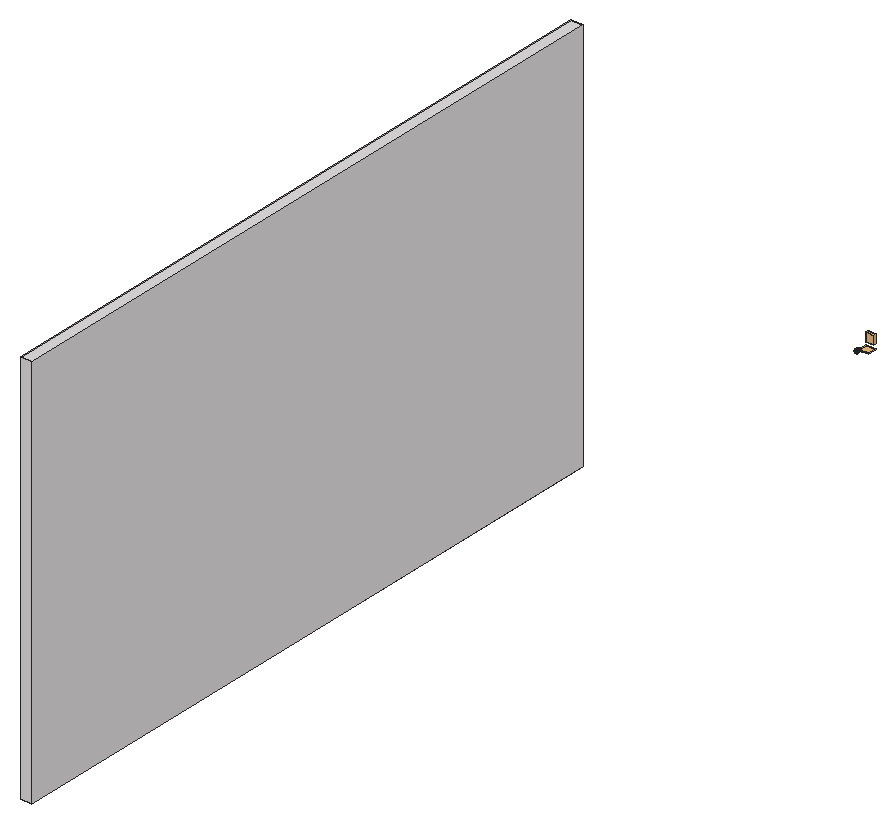
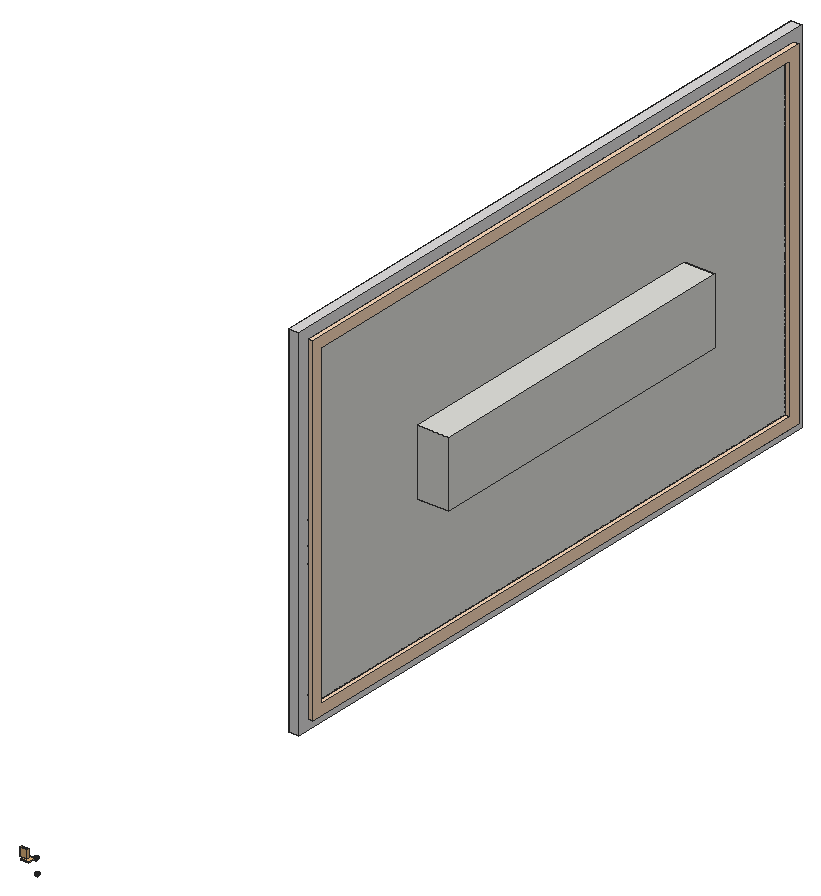
# SketchUp Ruby script. Lengths in inches.
U = 1.inch
M = Sketchup.active_model
def pt(a) = Geom::Point3d.new(a.map { |v| v * U })
def face(e, loops, mat)
  f = e.add_face(loops[0].map { |a| pt(a) })
  loops[1..].each { |l| e.add_face(l.map { |a| pt(a) }).erase! }
  f.material = f.back_material = mat if mat
  f
end
# faces: each face lists its corners as indices into pts; further lists are holes
def faces(e, pts, list, mat = nil) = list.each { |f| face(e, (f[0].is_a?(Array) ? f : [f]).map { |l| l.map { |i| pts[i] } }, mat) }
# xy, xz, yz: faces in a plane at the given z, y or x. An outline is a flat list of corners, or four numbers for a rectangle; further outlines are holes
def ring(l) = l.size == 4 ? [[l[0], l[1]], [l[2], l[1]], [l[2], l[3]], [l[0], l[3]]] : l.each_slice(2).to_a
def flat(e, list, mat, &to3) = list.each { |f| face(e, (f[0].is_a?(Array) ? f : [f]).map { |l| ring(l).map { |u, v| to3.(u, v) } }, mat) }
def xy(e, z, list, mat = nil) = flat(e, list, mat) { |x, y| [x, y, z] }
def xz(e, y, list, mat = nil) = flat(e, list, mat) { |x, z| [x, y, z] }
def yz(e, x, list, mat = nil) = flat(e, list, mat) { |y, z| [x, y, z] }
def lines(e, pts, list) = list.each { |a, b| e.add_line(pt(pts[a]), pt(pts[b])) }
# prism: a flat outline (further loops are holes) pulled along v
def prism(e, loops, v, mat = nil)
  f = face(e, loops, mat); d = Geom::Vector3d.new(v.map { |x| x * U })
  f.pushpull(f.normal.samedirection?(d) ? d.length : -d.length)
end
def box(e, o, s, mat = nil) = prism(e, [[o, [o[0] + s[0], o[1], o[2]], [o[0] + s[0], o[1] + s[1], o[2]], [o[0], o[1] + s[1], o[2]]]], [0, 0, s[2]], mat)
def at(x, y, z, deg = 0) = Geom::Transformation.translation(pt([x, y, z])) * Geom::Transformation.rotation(ORIGIN, Z_AXIS, deg.degrees)
def axes(o, x, y, z) = Geom::Transformation.new([*x, 0, *y, 0, *z, 0, *pt(o).to_a, 1])
def part(name) = M.definitions.add(name)
# library, detail: a bought-in or finely detailed component or shape, given as its bounding box
def library(name, o, s) = part(name).tap { |d| box(d.entities, o, s) }
def detail(e, o, s) = box(e.add_group.entities, o, s)
def put(e, d, t, mat = nil) = e.add_instance(d, t).tap { |i| i.material = mat if mat }
def group(e, t, mat = nil) = e.add_group.tap { |g| g.transformation = t; g.material = mat if mat }.entities
root = M.entities
M.materials.add("TV  BG light").color = [252, 218, 188]
M.materials.add("[Stone Vein Gray]").color = [225, 223, 223]
M.materials.add("green").color = [174, 139, 102]
M.materials.add("vio").color = [206, 114, 100]
c1 = part("3DGeom~250_Defintion")
p = [[-24.32,49.98,-496.93],[-31.18,-167.76,-459.32],[-244.86,-167.22,-390.18],[228.94,35.96,-443.61],[-244.86,-167.22,-390.18],[-271.06,50.6,-417.1],
  [208.38,242.18,-355.22],[-10.94,254.33,-401.4],[-271.06,50.6,-417.1],[208.38,242.18,-355.22],[-10.94,254.33,-401.4],[-29.68,-340.55,-298.625],
  [-153.05,-340.24,-258.71],[188.15,-179.91,-413.14],[-153.05,-340.24,-258.71],[-244.86,-167.22,-390.18],[420.85,12.3,-271.43],[374.59,221.7,-206.1],
  [374.59,221.7,-206.1],[208.38,242.18,-355.22],[-271.06,50.6,-417.1],[-395.65,-178.42,-224.25],[-445.17,37.67,-225.51],[-244.86,-167.22,-390.18],
  [-224.63,254.87,-332.26],[-10.94,254.33,-401.4],[-271.06,50.6,-417.1],[-224.63,254.87,-332.26],[96.95,-347.5625,-271.96],[354.35,-200.39,-264.02],
  [131.99,383.52,-171.65],[208.38,242.18,-355.22],[-10.94,254.33,-401.4],[5.36,390.53,-198.31],[-224.63,254.87,-332.26],[-240.11,-346.7,-162.91],
  [-153.05,-340.24,-258.71],[227.95,371.69,-85.56],[374.59,221.7,-206.1],[-224.63,254.87,-332.26],[-375.41,243.67,-166.34],[-118.01,390.84,-158.39],
  [-375.41,243.67,-166.34],[-153.05,-340.24,-258.71],[-29.68,-340.55,-298.625],[-20.23,-422.09,-57.92],[-29.68,-340.55,-298.625],[96.95,-347.5625,-271.96],
  [96.95,-347.5625,-271.96],[192.91,-359.39,-185.87],[192.91,-359.39,-185.87],[500,-14.65,-26.51],[354.35,-200.39,-264.02],[420.85,12.3,-271.43],
  [443.13,198.36,6],[420.85,12.3,-271.43],[420.85,12.3,-271.43],[374.59,221.7,-206.1],[422.9,-223.73,-51.92],[192.91,-359.39,-185.87],
  [354.35,-200.39,-264.02],[354.35,-200.39,-264.02],[-240.11,-346.7,-162.91],[-153.05,-340.24,-258.71],[-443.13,-198.36,-6],[-500,14.65,26.51],
  [-267.52,-358.22,-36.9],[267.52,358.22,36.9],[374.59,221.7,-206.1],[267.52,358.22,36.9],[374.59,221.7,-206.1],[227.95,371.69,-85.56],
  [20.23,422.09,57.92],[192.91,-359.39,-185.87],[232.48,-372.86,-63.41],[232.48,-372.86,-63.41],[192.91,-359.39,-185.87],[-422.9,223.73,51.92],
  [-205.0625,384.375,-62.6],[-375.41,243.67,-166.34],[-205.0625,384.375,-62.6],[-267.52,-358.22,-36.9],[-240.11,-346.7,-162.91],[267.52,358.22,36.9],
  [232.48,-372.86,-63.41],[205.0625,-384.375,62.6],[375.41,-243.67,166.34],[205.0625,-384.375,62.6],[-205.0625,384.375,-62.6],[-232.48,372.86,63.41],
  [-232.48,372.86,63.41],[-227.95,-371.69,85.56],[-267.52,-358.22,-36.9],[-131.99,-383.52,171.65],[-227.95,-371.69,85.56],[-5.36,-390.53,198.31],
  [205.0625,-384.375,62.6],[118.01,-390.84,158.39],[445.17,-37.67,225.51],[-227.95,-371.69,85.56],[395.65,178.42,224.25],[-374.59,-221.7,206.1],
  [240.11,346.7,162.91],[240.11,346.7,162.91],[267.52,358.22,36.9],[-420.85,-12.3,271.43],[240.11,346.7,162.91],[-354.35,200.39,264.02],
  [-232.48,372.86,63.41],[153.05,340.24,258.71],[29.68,340.55,298.625],[-96.95,347.5625,271.96],[-192.91,359.39,185.87],[224.63,-254.87,332.26],
  [205.0625,-384.375,62.6],[224.63,-254.87,332.26],[205.0625,-384.375,62.6],[375.41,-243.67,166.34],[-232.48,372.86,63.41],[-192.91,359.39,185.87],
  [-374.59,-221.7,206.1],[-227.95,-371.69,85.56],[10.94,-254.33,401.4],[10.94,-254.33,401.4],[224.63,-254.87,332.26],[153.05,340.24,258.71],
  [240.11,346.7,162.91],[271.0625,-50.61,417.1],[224.63,-254.87,332.26],[-208.38,-242.18,355.22],[-374.59,-221.7,206.1],[-208.38,-242.18,355.22],
  [-192.91,359.39,185.87],[-354.35,200.39,264.02],[-188.15,179.91,413.14],[-192.91,359.39,185.87],[-96.95,347.5625,271.96],[-208.38,-242.18,355.22],
  [10.94,-254.33,401.4],[-420.85,-12.3,271.43],[-374.59,-221.7,206.1],[-208.38,-242.18,355.22],[244.86,167.22,390.18],[153.05,340.24,258.71],
  [29.68,340.55,298.625],[244.86,167.22,390.18],[153.05,340.24,258.71],[-354.35,200.39,264.02],[-420.85,-12.3,271.43],[-228.94,-35.96,443.61],
  [-354.35,200.39,264.02],[-420.85,-12.3,271.43],[-96.95,347.5625,271.96],[31.18,167.76,459.32],[-96.95,347.5625,271.96],[29.68,340.55,298.625],
  [29.68,340.55,298.625],[244.86,167.22,390.18],[24.32,-49.98,496.93],[10.94,-254.33,401.4],[224.63,-254.87,332.26],[224.63,-254.87,332.26],
  [271.0625,-50.61,417.1],[271.0625,-50.61,417.1],[244.86,167.22,390.18],[271.0625,-50.61,417.1]]
faces(c1.entities,p,[[0,1,2],[3,1,0],[0,4,5],[6,3,0],[7,0,8],[9,0,10],[1,11,12],[13,11,1],
  [1,14,15],[3,13,1],[16,13,3],[17,16,3],[18,3,19],[20,21,22],[20,23,21],[24,20,22],
  [25,26,27],[13,28,11],[29,28,13],[16,29,13],[30,31,32],[33,32,34],[30,32,33],[23,35,21],
  [23,36,35],[37,38,31],[37,31,30],[39,22,40],[41,34,42],[33,34,41],[43,44,45],[46,47,45],
  [48,49,45],[29,50,28],[51,52,53],[54,51,55],[54,56,57],[58,59,60],[51,58,61],[62,63,45],
  [22,64,65],[22,21,64],[40,22,65],[21,66,64],[21,35,66],[67,54,68],[69,70,71],[30,33,72],
  [33,41,72],[73,74,45],[58,75,76],[37,30,72],[40,65,77],[78,40,77],[41,79,80],[81,82,45],
  [41,80,72],[83,37,72],[84,85,45],[86,87,75],[86,75,58],[88,77,89],[80,90,72],[91,92,45],
  [93,94,45],[95,93,45],[96,97,45],[97,95,45],[98,86,58],[98,58,51],[64,66,99],[100,98,51],
  [100,51,54],[64,99,101],[65,64,101],[102,100,54],[103,54,104],[65,101,105],[77,65,105],[106,83,72],
  [77,105,107],[108,77,107],[109,106,72],[110,109,72],[111,110,72],[112,111,72],[90,112,72],[113,97,114],
  [115,116,117],[118,107,119],[120,121,93],[122,95,97],[123,97,124],[125,100,126],[127,128,86],[127,86,98],
  [129,93,95],[130,93,131],[132,133,134],[135,134,136],[137,95,138],[139,140,141],[142,98,100],[143,142,100],
  [142,127,98],[144,145,146],[147,148,149],[150,149,134],[151,141,149],[152,134,153],[154,153,155],[156,153,157],
  [158,159,160],[158,161,162],[149,141,159],[153,163,164],[149,159,158],[134,149,158],[134,158,153],[153,158,165]],"vio")
c2 = library("3DGeom~185_Defintion",[-474.17,-47.42,-500],[948.34,94.84,1000])
c3 = part("3DGeom~186_Defintion")
p = [[474.17,30.45,-478.03],[446.82,25.72,-499.58],[445.25,33.625,-500],[474.17,30.45,-478.03],[445.25,33.625,-500],[447.56,41.1,-497.47],
  [474.17,30.45,-478.03],[451.84,19.51,-496.34],[446.82,25.72,-499.58],[474.17,30.45,-478.03],[447.56,41.1,-497.47],[453.12,46.15,-492.68],
  [474.17,30.45,-478.03],[458.97,16.66,-491.125],[451.84,19.51,-496.34],[474.17,30.45,-478.03],[453.12,46.15,-492.68],[460.45,47.42,-486.91],
  [474.17,30.45,-478.03],[466.3,17.93,-485.35],[458.97,16.66,-491.125],[474.17,30.45,-478.03],[460.45,47.42,-486.91],[467.58,44.57,-481.7],
  [474.17,30.45,-478.03],[471.87,22.98,-480.56],[466.3,17.93,-485.35],[474.17,30.45,-478.03],[467.58,44.57,-481.7],[472.6,38.36,-478.45],
  [-471.62,-44.41,472.73],[-461.42,-33.9375,500],[-474.17,-30.14,466.08],[-471.62,-44.41,472.73],[-474.17,-30.14,466.08],[-473.6875,-38.09,467.3],
  [-474.17,-30.14,466.08],[-461.42,-33.9375,500],[-470.35,-17.77,476.39],[-474.17,-30.14,466.08],[-470.35,-17.77,476.39],[-472.95,-22.71,469.41],
  [-465.24,-46.31,489.69],[-471.62,-44.41,472.73],[-468.53,-47.42,480.93],[-465.24,-46.31,489.69],[-461.42,-33.9375,500],[-471.62,-44.41,472.73],
  [-470.35,-17.77,476.39],[-461.42,-33.9375,500],[-463.97,-19.67,493.35],[-470.35,-17.77,476.39],[-463.97,-19.67,493.35],[-467.06,-16.66,485.15],
  [-461.42,-33.9375,500],[-465.24,-46.31,489.69],[-462.64,-41.37,496.67],[-461.42,-33.9375,500],[-461.9,-25.99,498.78],[-463.97,-19.67,493.35]]
faces(c3.entities,p,[[0,1,2],[3,4,5],[6,7,8],[9,10,11],[12,13,14],[15,16,17],[18,19,20],[21,22,23],
  [24,25,26],[27,28,29],[30,31,32],[33,34,35],[36,37,38],[39,40,41],[42,43,44],[45,46,47],
  [48,49,50],[51,52,53],[54,55,56],[57,58,59]],"green")
c4 = part("3DGeom~220_Defintion")
p = [[-57.64,36.25,-500],[-74.66,-181.39,-451.57],[-284.21,-169.14,-366.97],[199.77,12.4,-463.71],[-284.21,-169.14,-366.97],[-299.61,50.39,-402.32],
  [197.74,223.52,-383.03],[-25.18,244.18,-414.46],[-299.61,50.39,-402.32],[-25.18,244.18,-414.46],[148.26,-202.04,-420.14],[403.65,-14.77,-303.17],
  [374.3125,199.99,-244],[374.3125,199.99,-244],[-71.68,-350.42,-282.14],[-192.66,-343.35,-233.3],[-192.66,-343.35,-233.3],[-284.21,-169.14,-366.97],
  [57.03,-362.35,-264],[324.83,-225.57,-281.11],[-25.18,244.18,-414.46],[-299.61,50.39,-402.32],[-234.73,256.42,-329.86],[142.74,374.75,-199.71],
  [-25.18,244.18,-414.46],[14.03,386.67,-217.86],[-25.18,244.18,-414.46],[-234.73,256.42,-329.86],[142.74,374.75,-199.71],[-25.18,244.18,-414.46],
  [14.03,386.67,-217.86],[-299.61,50.39,-402.32],[-284.21,-169.14,-366.97],[-424.23,-168.6,-189.02],[-461.29,51.02,-196.83],[-234.73,256.42,-329.86],
  [244.68,361.16,-119.44],[374.3125,199.99,-244],[197.74,223.52,-383.03],[197.74,223.52,-383.03],[142.74,374.75,-199.71],[-192.66,-343.35,-233.3],
  [-273.5,-343.04,-130.56],[-234.73,256.42,-329.86],[-374.75,256.97,-151.9],[-106.95,393.74,-169.02],[-374.75,256.97,-151.9],[499.375,-37.98,-61.39],
  [324.83,-225.57,-281.11],[403.65,-14.77,-303.17],[457.21,179.89,-34.61],[403.65,-14.77,-303.17],[403.65,-14.77,-303.17],[374.3125,199.99,-244],
  [-192.66,-343.35,-233.3],[-71.68,-350.42,-282.14],[-49.48,-425.5625,-37.11],[-71.68,-350.42,-282.14],[57.03,-362.35,-264],[158.97,-375.93,-183.73],
  [407.73,-245.68,-71.73],[158.97,-375.93,-183.73],[324.83,-225.57,-281.11],[407.73,-245.68,-71.73],[324.83,-225.57,-281.11],[57.03,-362.35,-264],
  [158.97,-375.93,-183.73],[292.54,349.56,1.44],[374.3125,199.99,-244],[292.54,349.56,1.44],[374.3125,199.99,-244],[244.68,361.16,-119.44],
  [-273.5,-343.04,-130.56],[-192.66,-343.35,-233.3],[49.48,425.5625,37.11],[-457.21,-179.89,34.61],[-499.375,37.98,61.39],[-374.75,256.97,-151.9],
  [-292.54,-349.56,-1.44],[158.97,-375.93,-183.73],[206.83,-387.54,-62.84],[407.73,-245.68,-71.73],[158.97,-375.93,-183.73],[-187.79,394.06,-66.27],
  [-374.75,256.97,-151.9],[-407.73,245.68,71.73],[-407.73,245.68,71.73],[-292.54,-349.56,-1.44],[-273.5,-343.04,-130.56],[292.54,349.56,1.44],
  [374.75,-256.97,151.9],[407.73,-245.68,-71.73],[461.29,-51.02,196.83],[374.75,-256.97,151.9],[-206.83,387.54,62.84],[187.79,-394.06,66.27],
  [374.75,-256.97,151.9],[424.23,168.6,189.02],[-244.68,-361.16,119.44],[-292.54,-349.56,-1.44],[-142.74,-374.75,199.71],[-14.03,-386.67,217.86],
  [106.95,-393.74,169.02],[273.5,343.04,130.56],[273.5,343.04,130.56],[292.54,349.56,1.44],[-244.68,-361.16,119.44],[273.5,343.04,130.56],
  [-244.68,-361.16,119.44],[-374.3125,-199.99,244],[-374.3125,-199.99,244],[192.66,343.35,233.3],[71.68,350.42,282.14],[-57.03,362.35,264],
  [-158.97,375.93,183.73],[-374.3125,-199.99,244],[-403.65,14.77,303.17],[-407.73,245.68,71.73],[-403.65,14.77,303.17],[-324.83,225.57,281.11],
  [-324.83,225.57,281.11],[234.73,-256.42,329.86],[234.73,-256.42,329.86],[374.75,-256.97,151.9],[-407.73,245.68,71.73],[-403.65,14.77,303.17],
  [-324.83,225.57,281.11],[-374.3125,-199.99,244],[192.66,343.35,233.3],[273.5,343.04,130.56],[299.61,-50.39,402.32],[234.73,-256.42,329.86],
  [25.18,-244.18,414.46],[25.18,-244.18,414.46],[234.73,-256.42,329.86],[-158.97,375.93,183.73],[-324.83,225.57,281.11],[-148.26,202.04,420.14],
  [-158.97,375.93,183.73],[-57.03,362.35,264],[284.21,169.14,366.97],[192.66,343.35,233.3],[-197.74,-223.52,383.03],[-142.74,-374.75,199.71],
  [-14.03,-386.67,217.86],[-374.3125,-199.99,244],[-197.74,-223.52,383.03],[-14.03,-386.67,217.86],[25.18,-244.18,414.46],[71.68,350.42,282.14],
  [284.21,169.14,366.97],[192.66,343.35,233.3],[-403.65,14.77,303.17],[-374.3125,-199.99,244],[-57.03,362.35,264],[74.66,181.39,451.57],
  [-57.03,362.35,264],[71.68,350.42,282.14],[-199.77,-12.4,463.71],[71.68,350.42,282.14],[284.21,169.14,366.97],[57.64,-36.25,500],
  [234.73,-256.42,329.86],[234.73,-256.42,329.86],[299.61,-50.39,402.32],[299.61,-50.39,402.32],[284.21,169.14,366.97],[299.61,-50.39,402.32]]
faces(c4.entities,p,[[0,1,2],[3,1,0],[0,4,5],[6,3,0],[7,0,8],[6,0,9],[3,10,1],[11,10,3],
  [12,11,3],[13,3,6],[1,14,15],[10,14,1],[1,16,17],[10,18,14],[19,18,10],[11,19,10],
  [20,21,22],[23,6,24],[25,26,27],[28,29,30],[31,32,33],[31,33,34],[35,31,34],[36,37,38],
  [36,39,40],[32,41,42],[32,42,33],[43,34,44],[45,27,46],[25,27,45],[47,48,49],[50,47,51],
  [50,52,53],[54,55,56],[57,58,56],[19,59,18],[60,61,62],[47,63,64],[65,66,56],[67,50,68],
  [69,70,71],[72,73,56],[40,25,74],[25,45,74],[36,40,74],[34,75,76],[34,33,75],[77,34,76],
  [33,78,75],[33,42,78],[79,80,56],[81,80,82],[45,46,83],[45,83,74],[84,76,85],[83,46,86],
  [87,88,56],[89,36,74],[90,80,91],[92,93,63],[92,63,47],[83,86,94],[83,94,74],[80,95,56],
  [96,95,80],[97,92,47],[97,47,50],[98,99,56],[100,98,56],[101,100,56],[95,102,56],[102,101,56],
  [103,97,50],[104,50,105],[75,78,106],[107,89,74],[75,108,109],[76,75,110],[111,107,74],[112,111,74],
  [113,112,74],[114,113,74],[94,114,74],[76,115,116],[117,76,118],[94,86,119],[94,120,114],[121,102,95],
  [122,95,123],[124,125,126],[127,98,100],[128,97,129],[130,131,93],[130,93,92],[132,101,102],[133,102,134],
  [135,136,137],[138,137,139],[140,92,97],[141,140,97],[140,130,92],[142,143,144],[145,100,146],[142,147,148],
  [149,150,151],[152,153,142],[154,137,155],[156,155,157],[136,152,158],[136,158,137],[159,155,160],[152,142,158],
  [161,148,162],[161,163,164],[155,165,166],[158,142,148],[155,161,167],[158,148,161],[137,158,161],[137,161,155]],"vio")
c5 = library("3DGeom~171_Defintion",[-163.52,-500,-478.3],[327.04,1000,956.6])
c6 = part("3DGeom~172_Defintion")
p = [[-160.83,493.0625,-454.31],[-133.02,479.16,-476.94],[-143.16,476.9375,-478.3],[-160.83,493.0625,-454.31],[-153.32,477.81,-475.6],[-160.83,493.0625,-454.31],
  [-125.62,483.875,-471.85],[-160.83,493.0625,-454.31],[-153.32,477.81,-475.6],[-160.77,481.53,-469.53],[-160.83,493.0625,-454.31],[-122.93,489.82,-464.42],
  [-125.62,483.875,-471.85],[-160.83,493.0625,-454.31],[-160.77,481.53,-469.53],[-163.52,487.11,-461.74],[-160.83,493.0625,-454.31],[-125.68,495.41,-456.63],
  [-122.93,489.82,-464.42],[-160.83,493.0625,-454.31],[-133.13,499.13,-450.57],[-125.68,495.41,-456.63],[-160.83,493.0625,-454.31],[-153.43,497.78,-449.23],
  [-143.29,500,-447.86],[-160.83,493.0625,-454.31],[-143.29,500,-447.86],[-133.13,499.13,-450.57],[160.33,-486.4,444.8],[144.67,-497.09,441.27],
  [153.43,-492.12,440.5],[144.67,-497.09,441.27],[132.66,-492.22,474],[130.84,-500,455.87],[144.67,-497.09,441.27],[130.84,-500,455.87],
  [136.4,-499.97,446.89],[160.33,-486.4,444.8],[132.66,-492.22,474],[144.67,-497.09,441.27],[162.15,-478.62,462.94],[132.66,-492.22,474],
  [160.33,-486.4,444.8],[162.15,-478.62,462.94],[160.33,-486.4,444.8],[163.52,-481.46,453.02],[132.66,-492.22,474],[129.47,-497.16,465.79],
  [130.84,-500,455.87],[148.32,-481.53,477.54],[132.66,-492.22,474],[162.15,-478.62,462.94],[148.32,-481.53,477.54],[162.15,-478.62,462.94],
  [156.59,-478.65,471.92],[132.66,-492.22,474],[148.32,-481.53,477.54],[139.5625,-486.5,478.3]]
faces(c6.entities,p,[[0,1,2],[3,2,4],[5,6,1],[7,8,9],[10,11,12],[13,14,15],[16,17,18],[19,20,21],
  [22,23,24],[25,26,27],[28,29,30],[31,32,33],[34,35,36],[37,38,39],[40,41,42],[43,44,45],
  [46,47,48],[49,50,51],[52,53,54],[55,56,57]],"green")
g1 = group(root,at(6,30.44,133.8))
xy(g1,-98.8,[[3,18,4,77.56]],"[Stone Vein Gray]")
xy(g1,-84.8,[[0,32,3,63.56]])
xy(g1,-78.55,[[0,32,3,63.56]])
xy(g1,-64.55,[[3,18,4,77.56]],"[Stone Vein Gray]")
xz(g1,18,[[3,-98.8,4,-64.55]],"[Stone Vein Gray]")
xz(g1,32,[[0,-84.8,3,-78.55]])
xz(g1,63.56,[[0,-84.8,3,-78.55]])
xz(g1,77.56,[[3,-98.8,4,-64.55]],"[Stone Vein Gray]")
yz(g1,0,[[32,-84.8,63.56,-78.55]])
yz(g1,3,[[[20,-96.8,75.56,-66.55],[32,-84.8,63.56,-78.55]]])
yz(g1,3,[[[18,-98.8,77.56,-64.55],[19,-97.8,76.56,-65.55]]],"[Stone Vein Gray]")
yz(g1,4,[[18,-98.8,77.56,-64.55]],"[Stone Vein Gray]")
g2 = group(g1,at(3,19,-97.8),"TV  BG light")
prism(g2,[[[-0.5,0,32.25],[-0.5,57.56,32.25],[-0.5,57.56,0],[-0.5,0,0]],[[-0.5,56.56,31.25],[-0.5,1,31.25],[-0.5,1,1],[-0.5,56.56,1]]],[0.5,0,0])
g3 = group(root,at(15.3125,134.49,26.21))
put(g3,c1,axes([-1.72,-1.11,7.9375],[0,0.00039,0],[0,0,-0.00039],[-0.00039,0,0]),"vio")
g4 = group(root,at(15.3125,134.49,26.21))
put(g4,c2,axes([-1.3,-0.69,7.91],[0,0.00081,0],[0,0,-0.00081],[-0.00081,0,0]),"green")
put(g4,c3,axes([-1.3,-0.69,7.91],[0,0.00081,0],[0,0,-0.00081],[-0.00081,0,0]),"green")
g5 = group(root,at(15.3125,134.49,26.21))
put(g5,c4,axes([-2.5,-0.29,7.23],[0,0.00039,0],[0,0,-0.00039],[-0.00039,0,0]),"vio")
g6 = group(root,at(15.3125,134.49,26.21))
put(g6,c5,axes([-1.3,-0.26,8.65],[0,0.00073,0],[0,0,-0.00073],[-0.00073,0,0]),"green")
put(g6,c6,axes([-1.3,-0.26,8.65],[0,0.00073,0],[0,0,-0.00073],[-0.00073,0,0]),"green")
